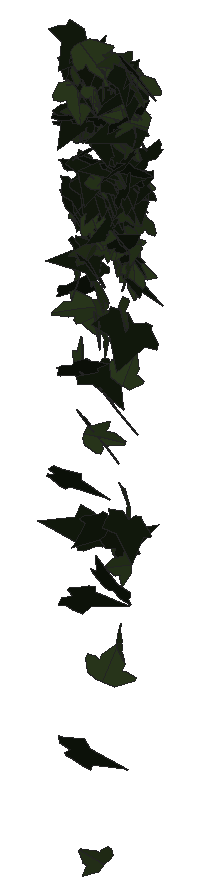
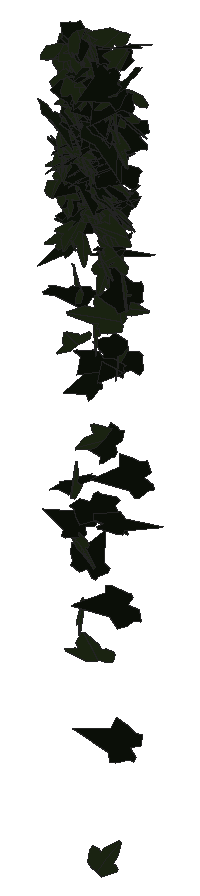
# SketchUp Ruby script. Lengths in inches.
U = 1.inch
M = Sketchup.active_model
def pt(a) = Geom::Point3d.new(a.map { |v| v * U })
def face(e, loops, mat)
  f = e.add_face(loops[0].map { |a| pt(a) })
  loops[1..].each { |l| e.add_face(l.map { |a| pt(a) }).erase! }
  f.material = f.back_material = mat if mat
  f
end
# faces: each face lists its corners as indices into pts; further lists are holes
def faces(e, pts, list, mat = nil) = list.each { |f| face(e, (f[0].is_a?(Array) ? f : [f]).map { |l| l.map { |i| pts[i] } }, mat) }
# xy, xz, yz: faces in a plane at the given z, y or x. An outline is a flat list of corners, or four numbers for a rectangle; further outlines are holes
def ring(l) = l.size == 4 ? [[l[0], l[1]], [l[2], l[1]], [l[2], l[3]], [l[0], l[3]]] : l.each_slice(2).to_a
def flat(e, list, mat, &to3) = list.each { |f| face(e, (f[0].is_a?(Array) ? f : [f]).map { |l| ring(l).map { |u, v| to3.(u, v) } }, mat) }
def xy(e, z, list, mat = nil) = flat(e, list, mat) { |x, y| [x, y, z] }
def xz(e, y, list, mat = nil) = flat(e, list, mat) { |x, z| [x, y, z] }
def yz(e, x, list, mat = nil) = flat(e, list, mat) { |y, z| [x, y, z] }
def lines(e, pts, list) = list.each { |a, b| e.add_line(pt(pts[a]), pt(pts[b])) }
# prism: a flat outline (further loops are holes) pulled along v
def prism(e, loops, v, mat = nil)
  f = face(e, loops, mat); d = Geom::Vector3d.new(v.map { |x| x * U })
  f.pushpull(f.normal.samedirection?(d) ? d.length : -d.length)
end
def box(e, o, s, mat = nil) = prism(e, [[o, [o[0] + s[0], o[1], o[2]], [o[0] + s[0], o[1] + s[1], o[2]], [o[0], o[1] + s[1], o[2]]]], [0, 0, s[2]], mat)
def at(x, y, z, deg = 0) = Geom::Transformation.translation(pt([x, y, z])) * Geom::Transformation.rotation(ORIGIN, Z_AXIS, deg.degrees)
def axes(o, x, y, z) = Geom::Transformation.new([*x, 0, *y, 0, *z, 0, *pt(o).to_a, 1])
def part(name) = M.definitions.add(name)
# library, detail: a bought-in or finely detailed component or shape, given as its bounding box
def library(name, o, s) = part(name).tap { |d| box(d.entities, o, s) }
def detail(e, o, s) = box(e.add_group.entities, o, s)
def put(e, d, t, mat = nil) = e.add_instance(d, t).tap { |i| i.material = mat if mat }
def group(e, t, mat = nil) = e.add_group.tap { |g| g.transformation = t; g.material = mat if mat }.entities
root = M.entities
M.materials.add("1026 AP 7946 SUNNY SIDE UP").color = [254, 231, 186]
M.materials.add("efeu1").color = [18, 25, 13]
M.materials.add("efeu2").color = [43, 57, 29]
c1 = part("ivyleaf_10")
p = [[0,0.5,-0.03],[-0.0625,2.02,-0.43],[-0.19,2.01,-0.46],[-0.54,1.05,-0.29],[-0.52,0.625,-0.18],[-0.83,0.76,-0.28],
  [-1.16,0.64,-0.33],[-1.15,0.33,-0.24],[-0.77,-0.39,0.02],[-0.3,-0.51,0.16],[0.04,-0.48,0.23],[-0.02,2.01,-0.4375],
  [-0.06,2.01,-0.43],[0.04,-0.49,0.23],[0.67,-0.49,0.14],[1.38,0.36,-0.2],[1.375,0.51,-0.24],[0.81,0.65,-0.19],
  [0.62,0.59,-0.15],[0.6,1.09,-0.28],[0.5,1.23,-0.31]]
faces(c1.entities,p,[[0,1,2,3,4,5,6,7,8,9,10],[11,12,0,13,14,15,16,17,18,19,20]],"efeu2")
c2 = part("ivyleaf_9")
p = [[1.54,2.16,1.25],[1.36,2.04,1.19],[-0.21,0.99,0.68],[-0.71,1.11,0.82],[-0.85,0.86,0.67],[-0.8,0.17,0.21],
  [-0.9,-0.01,0.1],[-0.67,-0.16,-0.02],[-0.08,-0.08,-0.05],[-0.03,-0.6,-0.4],[0.65,-0.88,-0.66],[0.83,-0.6,-0.49],
  [1.29,-0.42,-0.43],[1.8125,-0.07,-0.26],[1.21,0.44,0.15]]
faces(c2.entities,p,[[0,1,2,3,4,5,6,7,8,9,10,11,12,13,14]],"efeu1")
put(root,c1,axes([113.11,212.68,263.1],[0.14339,-0.21854,-0.11555],[-0.02528,0.11276,-0.24183],[0.38453,0.08891,0.02719]),"1026 AP 7946 SUNNY SIDE UP")
put(root,c1,axes([113.16,212.9,266.08],[0.28745,-0.13177,-0.11438],[-0.11976,0.0822,-0.23077],[0.24219,0.19704,0.02164]),"1026 AP 7946 SUNNY SIDE UP")
put(root,c1,axes([113.23,212.76,262.51],[-0.08031,-0.00401,0.24324],[-0.13938,-0.2236,-0.02498],[0.3442,-0.09148,0.04664]),"1026 AP 7946 SUNNY SIDE UP")
put(root,c2,axes([112.91,212.79,267.24],[0.15405,-0.23556,0.00086],[-0.00345,-0.00327,-0.26283],[0.3704,0.09794,-0.00281]),"1026 AP 7946 SUNNY SIDE UP")
put(root,c2,axes([112.79,212.7,266.14],[0.27707,-0.02474,0.18756],[0.28605,0.06019,-0.17247],[-0.04208,0.24622,0.06254]),"1026 AP 7946 SUNNY SIDE UP")
put(root,c2,axes([113.15,212.73,266.41],[-0.35367,-0.0146,-0.10812],[0.16648,-0.03342,-0.22934],[-0.00163,-0.24591,0.03612]),"1026 AP 7946 SUNNY SIDE UP")
put(root,c2,axes([112.97,212.71,262.75],[0.24374,0.17951,0.06208],[-0.08387,-0.03196,0.24337],[0.28515,-0.16284,0.01852]),"1026 AP 7946 SUNNY SIDE UP")
put(root,c2,axes([112.83,212.51,259.08],[0.31998,-0.00455,0.13415],[0.204,-0.01583,-0.20949],[0.01944,0.24109,-0.00981]),"1026 AP 7946 SUNNY SIDE UP")
put(root,c1,axes([113.1875,212.68,261.35],[-0.03383,0.16262,-0.1746],[-0.02819,0.16949,0.16995],[0.36931,0.02784,-0.00302]),"1026 AP 7946 SUNNY SIDE UP")
put(root,c2,axes([113.16,212.82,267.87],[-0.27569,-0.18209,0.07565],[0.01248,-0.10621,-0.24894],[0.30908,-0.15813,0.07752]),"1026 AP 7946 SUNNY SIDE UP")
put(root,c2,axes([112.98,212.79,264.84],[0.09227,-0.24022,0.02704],[0.00198,-0.02811,-0.25485],[0.3802,0.05844,-0.00524]),"1026 AP 7946 SUNNY SIDE UP")
put(root,c1,axes([113.11,212.9,266.38],[0.14453,-0.21357,0.09729],[0.10596,-0.07425,-0.23795],[0.35238,0.10992,0.03165]),"1026 AP 7946 SUNNY SIDE UP")
put(root,c2,axes([113.46,212.74,258.04],[-0.20765,0.00261,0.22035],[-0.33108,-0.04579,-0.13363],[0.05915,-0.24716,0.02559]),"1026 AP 7946 SUNNY SIDE UP")
put(root,c1,axes([112.89,213.01,264.22],[0.07986,0.02033,0.23675],[0.36249,-0.01001,-0.05166],[0.00854,0.23503,-0.02129]),"1026 AP 7946 SUNNY SIDE UP")
put(root,c2,axes([112.98,212.7,264.55],[0.15702,-0.21785,0.07841],[0.03027,-0.07613,-0.24693],[0.36223,0.10079,-0.01335]),"1026 AP 7946 SUNNY SIDE UP")
put(root,c2,axes([113.44,212.88,264.79],[-0.16271,0.20616,0.07975],[-0.13387,0.0401,-0.2305],[-0.31864,-0.12212,0.05612]),"1026 AP 7946 SUNNY SIDE UP")
put(root,c2,axes([112.97,212.79,256.57],[0.08033,0.09459,-0.23035],[0.13195,0.20812,0.11141],[0.35906,-0.09764,0.01059]),"1026 AP 7946 SUNNY SIDE UP")
put(root,c1,axes([112.95,212.97,264.47],[0.23372,-0.06389,-0.18259],[0.28207,-0.01951,0.16245],[-0.08877,-0.23021,0.03545]),"1026 AP 7946 SUNNY SIDE UP")
put(root,c1,axes([113.15,212.92,266.87],[0.02845,0.25366,0.00702],[-0.0002,0.00539,-0.26195],[-0.39894,0.01809,0.00063]),"1026 AP 7946 SUNNY SIDE UP")
put(root,c2,axes([113.38,212.6875,264.37],[0.02959,0.08398,0.26584],[-0.10849,0.25116,-0.0777],[-0.41194,-0.06012,0.03956]),"1026 AP 7946 SUNNY SIDE UP")
put(root,c2,axes([113.19,212.9375,264.66],[-0.15171,-0.21094,0.06917],[-0.00318,-0.07369,-0.23769],[0.34865,-0.09246,0.02793]),"1026 AP 7946 SUNNY SIDE UP")
put(root,c2,axes([113.17,212.8125,266.98],[0.25403,0.19503,0.04641],[0.05454,0.0283,-0.26059],[-0.30959,0.16502,-0.00783]),"1026 AP 7946 SUNNY SIDE UP")
put(root,c1,axes([113.1,212.65,266.89],[0.39992,0.05938,0.06721],[0.10794,-0.0098,-0.26794],[-0.0865,0.2623,-0.02361]),"1026 AP 7946 SUNNY SIDE UP")
put(root,c2,axes([112.99,213.12,259.95],[0.24103,-0.18315,0.08435],[0.07013,-0.0707,-0.24622],[0.30826,0.1593,-0.00994]),"1026 AP 7946 SUNNY SIDE UP")
put(root,c1,axes([113.3,212.78,266.48],[-0.32134,-0.14247,0.01436],[-0.0011,-0.0247,-0.25598],[0.22522,-0.2034,0.01923]),"1026 AP 7946 SUNNY SIDE UP")
put(root,c2,axes([113.08,212.6875,265.43],[0.34831,0.10374,0.05498],[0.08308,0.01148,-0.25163],[-0.16307,0.22743,-0.01077]),"1026 AP 7946 SUNNY SIDE UP")
put(root,c2,axes([113.16,212.86,267.14],[0.16056,0.15054,0.22448],[0.19108,0.17984,-0.18634],[-0.36878,0.15872,0.00118]),"1026 AP 7946 SUNNY SIDE UP")
put(root,c1,axes([113.37,213.02,251.24],[-0.11316,-0.14568,-0.20001],[-0.16278,-0.16379,0.1659],[-0.34406,0.12541,-0.0127]),"1026 AP 7946 SUNNY SIDE UP")
put(root,c2,axes([113.51,212.76,263.55],[-0.2734,-0.02419,0.17293],[-0.2298,-0.10097,-0.17139],[0.13573,-0.21969,0.05816]),"1026 AP 7946 SUNNY SIDE UP")
put(root,c1,axes([113.27,212.54,267.52],[0.03286,0.20384,0.17846],[-0.05247,0.17324,-0.20623],[-0.41615,-0.00575,0.04009]),"1026 AP 7946 SUNNY SIDE UP")
put(root,c2,axes([113.47,212.88,266.04],[-0.00762,0.24899,0.03723],[-0.09424,0.03258,-0.24913],[-0.3839,-0.01294,0.06042]),"1026 AP 7946 SUNNY SIDE UP")
put(root,c2,axes([113.125,212.71,263.75],[0.22541,-0.19566,-0.01982],[-0.02659,0.01007,-0.24969],[0.30782,0.14415,-0.00705]),"1026 AP 7946 SUNNY SIDE UP")
put(root,c1,axes([113.08,212.95,263.67],[0.2639,-0.02544,0.16899],[0.25765,-0.01316,-0.17474],[0.04311,0.23441,0.00992]),"1026 AP 7946 SUNNY SIDE UP")
put(root,c2,axes([113.46,212.7,265.86],[-0.03787,0.2489,-0.01265],[-0.00255,-0.01391,-0.25768],[-0.39196,-0.02396,0.0029]),"1026 AP 7946 SUNNY SIDE UP")
put(root,c2,axes([113.25,212.42,261.47],[0.25901,0.181,0.05835],[0.07257,0.03311,-0.25164],[-0.28875,0.17067,-0.01091]),"1026 AP 7946 SUNNY SIDE UP")
put(root,c1,axes([113.41,212.65,263.8],[-0.07233,-0.22693,0.05058],[-0.00303,-0.05099,-0.23869],[0.3655,-0.04533,0.00803]),"1026 AP 7946 SUNNY SIDE UP")
put(root,c1,axes([113.31,212.85,264.42],[-0.36001,-0.06725,-0.05867],[0.12713,-0.09934,-0.21603],[0.05415,-0.2139,0.11713]),"1026 AP 7946 SUNNY SIDE UP")
put(root,c1,axes([113.32,212.8125,266.36],[-0.02745,0.07669,-0.25279],[0.01927,-0.24585,-0.08135],[-0.40443,-0.01692,0.01328]),"1026 AP 7946 SUNNY SIDE UP")
put(root,c1,axes([113.42,212.85,265],[-0.36384,-0.07137,0.01785],[0.01596,-0.08896,-0.23302],[0.11453,-0.21434,0.08916]),"1026 AP 7946 SUNNY SIDE UP")
put(root,c2,axes([113.33,212.6,267.28],[-0.09798,-0.08593,0.25551],[0.2938,0.16522,0.10809],[-0.2909,0.19581,0.02311]),"1026 AP 7946 SUNNY SIDE UP")
put(root,c2,axes([113.35,212.9,265.01],[-0.28616,-0.08708,-0.14489],[0.2253,0.02007,-0.2044],[0.12866,-0.22882,0.03566]),"1026 AP 7946 SUNNY SIDE UP")
put(root,c2,axes([113.07,212.61,253.5625],[0.2214,-0.03551,0.22121],[0.31491,-0.07961,-0.14918],[0.13479,0.24431,-0.01485]),"1026 AP 7946 SUNNY SIDE UP")
put(root,c1,axes([113.48,212.94,265.11],[-0.03085,-0.24314,0.00966],[-0.00318,-0.01063,-0.25135],[0.38267,-0.01969,-0.00131]),"1026 AP 7946 SUNNY SIDE UP")
put(root,c1,axes([113.39,212.91,263.47],[0.23129,-0.17155,0.07394],[0.07233,-0.05639,-0.23312],[0.28393,0.15411,-0.00085]),"1026 AP 7946 SUNNY SIDE UP")
put(root,c1,axes([113.3125,212.89,259.88],[0.05431,0.06055,0.23759],[0.12432,0.21657,-0.06961],[-0.35316,0.08555,0.01203]),"1026 AP 7946 SUNNY SIDE UP")
put(root,c2,axes([113.55,212.78,266.6],[0.22399,0.15272,-0.1568],[-0.17696,-0.10415,-0.21556],[-0.29031,0.18132,0.01042]),"1026 AP 7946 SUNNY SIDE UP")
put(root,c2,axes([113.53,212.86,265.09],[-0.19793,0.10736,-0.18339],[0.15727,-0.15195,-0.16759],[-0.28748,-0.15704,0.03458]),"1026 AP 7946 SUNNY SIDE UP")
put(root,c2,axes([113.42,212.78,265.4],[-0.12178,-0.23438,0.06477],[-0.01196,-0.06502,-0.25433],[0.38192,-0.07677,0.01269]),"1026 AP 7946 SUNNY SIDE UP")
put(root,c2,axes([113.37,212.68,266.31],[0.34939,0.12801,0.00971],[0.02646,-0.01183,-0.26355],[-0.20001,0.22206,-0.0179]),"1026 AP 7946 SUNNY SIDE UP")
put(root,c1,axes([113.38,212.95,264.79],[0.31388,-0.09748,0.09918],[0.15047,-0.02389,-0.22817],[0.15502,0.22057,0.02067]),"1026 AP 7946 SUNNY SIDE UP")
put(root,c2,axes([113.54,212.79,265.05],[-0.31747,-0.10704,-0.08393],[0.14402,-0.00323,-0.23121],[0.15412,-0.21747,0.04316]),"1026 AP 7946 SUNNY SIDE UP")
put(root,c1,axes([113.5625,212.68,263.1],[-0.26868,0.17235,0.00308],[-0.02039,-0.01003,-0.24952],[-0.27025,-0.17059,0.01577]),"1026 AP 7946 SUNNY SIDE UP")
put(root,c1,axes([113.24,212.89,262.34],[0.06545,0.02044,0.28839],[0.39055,0.12888,-0.04701],[-0.20518,0.25184,0.00251]),"1026 AP 7946 SUNNY SIDE UP")
put(root,c1,axes([113.56,212.8,267.05],[-0.15315,0.19436,-0.13373],[-0.00695,-0.14327,-0.21657],[-0.36841,-0.07809,0.05968]),"1026 AP 7946 SUNNY SIDE UP")
put(root,c1,axes([113.52,212.81,267.05],[0.24578,0.19921,-0.01645],[0.00052,-0.02196,-0.2606],[-0.31439,0.1557,-0.01329]),"1026 AP 7946 SUNNY SIDE UP")
put(root,c1,axes([113.44,212.52,267.87],[0.17244,0.21559,0.12765],[0.11529,0.09997,-0.24792],[-0.37261,0.1307,-0.01763]),"1026 AP 7946 SUNNY SIDE UP")
put(root,c2,axes([113.54,212.8125,266.21],[0.35864,-0.0202,-0.10636],[-0.16272,-0.00034,-0.23572],[0.02872,0.25031,-0.00743]),"1026 AP 7946 SUNNY SIDE UP")
put(root,c2,axes([113.75,212.76,258.36],[0.02569,0.09211,-0.24125],[-0.04923,-0.23264,-0.09766],[-0.39339,0.03513,-0.00353]),"1026 AP 7946 SUNNY SIDE UP")
put(root,c2,axes([113.55,212.9375,265.17],[-0.09619,-0.23516,0.02652],[-0.00148,-0.02773,-0.2504],[0.3722,-0.06089,0.00586]),"1026 AP 7946 SUNNY SIDE UP")
put(root,c1,axes([113.75,212.73,264.03],[0.22627,-0.14545,-0.12574],[-0.15163,0.07474,-0.20987],[0.25622,0.17267,-0.01316]),"1026 AP 7946 SUNNY SIDE UP")
put(root,c1,axes([113.56,212.67,262.4],[-0.09415,0.15877,-0.17054],[0.07736,-0.15917,-0.17558],[-0.35331,-0.07716,0.007]),"1026 AP 7946 SUNNY SIDE UP")
put(root,c2,axes([113.75,212.84,265.09],[0.07144,0.23633,-0.03288],[-0.00345,-0.03345,-0.24808],[-0.37525,0.0453,-0.00398]),"1026 AP 7946 SUNNY SIDE UP")
put(root,c2,axes([113.51,212.78,261.39],[-0.12223,-0.12418,-0.20028],[0.22183,0.1358,-0.14721],[0.28581,-0.1585,0.02861]),"1026 AP 7946 SUNNY SIDE UP")
put(root,c1,axes([113.72,212.73,261.98],[0.16248,-0.18346,-0.14607],[-0.02925,0.14707,-0.21069],[0.36241,0.09412,0.04848]),"1026 AP 7946 SUNNY SIDE UP")
put(root,c1,axes([113.6,212.53,264.5],[0.13535,0.2368,0.0401],[0.03486,0.0319,-0.25918],[-0.37539,0.08834,-0.00961]),"1026 AP 7946 SUNNY SIDE UP")
put(root,c1,axes([113.71,212.91,264.65],[0.18507,-0.20631,0.01557],[-0.00186,-0.0194,-0.24456],[0.3254,0.11722,-0.01025]),"1026 AP 7946 SUNNY SIDE UP")
put(root,c1,axes([113.72,212.83,267.65],[0.19672,-0.23128,-0.00934],[0.00799,0.01156,-0.27063],[0.36379,0.12482,0.011]),"1026 AP 7946 SUNNY SIDE UP")
put(root,c2,axes([113.65,212.62,266.14],[0.23679,-0.08856,-0.18939],[-0.14171,0.17548,-0.16256],[0.28707,0.15967,0.07597]),"1026 AP 7946 SUNNY SIDE UP")
put(root,c1,axes([113.72,212.61,264.22],[0.29826,-0.16998,0.04957],[-0.02971,0.05208,0.26136],[-0.27661,-0.18888,0.02537]),"1026 AP 7946 SUNNY SIDE UP")
put(root,c1,axes([113.75,212.95,265.3125],[0.21138,-0.20333,0.02658],[0.03209,-0.0188,-0.25113],[0.32091,0.13581,0.00761]),"1026 AP 7946 SUNNY SIDE UP")
put(root,c1,axes([113.57,212.89,265.08],[0.30301,0.02641,0.15759],[0.24281,-0.01007,-0.19886],[-0.02261,0.24574,-0.02362]),"1026 AP 7946 SUNNY SIDE UP")
put(root,c1,axes([113.69,212.76,255.27],[0.38128,0.07194,-0.07632],[0.10061,0.04506,0.25966],[0.12803,-0.24964,0.02324]),"1026 AP 7946 SUNNY SIDE UP")
put(root,c2,axes([113.65,212.87,267],[-0.16687,-0.17968,-0.14989],[0.19049,0.09187,-0.20884],[0.30846,-0.15393,0.04788]),"1026 AP 7946 SUNNY SIDE UP")
put(root,c1,axes([113.88,212.93,263.75],[-0.29479,0.14058,0.04458],[-0.10442,-0.01972,-0.23485],[-0.20597,-0.19122,0.05525]),"1026 AP 7946 SUNNY SIDE UP")
put(root,c2,axes([113.83,212.78,257.03],[0.26502,-0.1448,0.12277],[-0.11692,0.09669,0.22836],[-0.2716,-0.18291,0.02149]),"1026 AP 7946 SUNNY SIDE UP")
put(root,c1,axes([113.86,212.86,267.36],[0.23774,-0.18729,-0.08885],[-0.07111,0.07287,-0.24733],[0.31561,0.1575,0.0112]),"1026 AP 7946 SUNNY SIDE UP")
put(root,c2,axes([113.67,212.94,265.03],[0.05691,-0.2404,0.01658],[0.00133,-0.01753,-0.25054],[0.379,0.03616,-0.00161]),"1026 AP 7946 SUNNY SIDE UP")
put(root,c2,axes([113.77,212.79,267.38],[-0.3007,-0.06196,-0.17097],[0.26485,0.0104,-0.20432],[0.0846,-0.25277,0.03193]),"1026 AP 7946 SUNNY SIDE UP")
put(root,c1,axes([113.81,212.81,266.78],[0.37204,-0.09439,-0.03052],[0.00008,0.07563,-0.25194],[0.15531,0.22607,0.07324]),"1026 AP 7946 SUNNY SIDE UP")
put(root,c2,axes([113.75,212.92,265.07],[-0.0422,-0.23813,0.05112],[0.0041,-0.05156,-0.24703],[0.38289,-0.02569,0.00828]),"1026 AP 7946 SUNNY SIDE UP")
put(root,c1,axes([113.85,212.9,265.14],[0.3407,-0.10555,-0.0133],[-0.03177,-0.01346,-0.24744],[0.16405,0.21661,-0.02029]),"1026 AP 7946 SUNNY SIDE UP")
put(root,c2,axes([113.74,212.9,265.3],[-0.02911,-0.24211,0.04988],[0.00429,-0.05013,-0.25036],[0.38864,-0.01758,0.0065]),"1026 AP 7946 SUNNY SIDE UP")
put(root,c1,axes([113.87,212.75,266.68],[-0.12507,0.23994,-0.03717],[-0.05429,-0.05017,-0.25597],[-0.37798,-0.07219,0.04906]),"1026 AP 7946 SUNNY SIDE UP")
put(root,c1,axes([113.79,212.83,267.38],[0.16912,-0.22218,0.0669],[0.12241,-0.03413,-0.24849],[0.34337,0.1216,0.05564]),"1026 AP 7946 SUNNY SIDE UP")
put(root,c2,axes([113.66,212.78,260.89],[0.30423,-0.14553,0.01707],[0.00407,-0.02541,-0.24882],[0.23043,0.19259,-0.01814]),"1026 AP 7946 SUNNY SIDE UP")
put(root,c1,axes([114.05,212.84,257.56],[0.1687,-0.13157,-0.18188],[-0.20295,0.12051,-0.17335],[0.27933,0.16702,-0.0161]),"1026 AP 7946 SUNNY SIDE UP")
put(root,c1,axes([113.83,212.61,265.375],[-0.27913,-0.15522,-0.06399],[0.15523,-0.02561,-0.22809],[0.21154,-0.18603,0.08293]),"1026 AP 7946 SUNNY SIDE UP")
put(root,c2,axes([113.74,212.88,265.13],[0.38046,0.02026,0.00087],[0.0015,-0.00267,-0.25014],[-0.03183,0.24195,-0.00141]),"1026 AP 7946 SUNNY SIDE UP")
put(root,c1,axes([113.97,212.89,266.89],[-0.22344,-0.20784,0.02095],[-0.00511,-0.02382,-0.25928],[0.32852,-0.14174,0.01022]),"1026 AP 7946 SUNNY SIDE UP")
put(root,c1,axes([113.97,212.87,267.54],[-0.29708,-0.17229,0.0156],[-0.00022,-0.02372,-0.26294],[0.2721,-0.18813,0.01682]),"1026 AP 7946 SUNNY SIDE UP")
put(root,c1,axes([113.96,212.84,267.76],[-0.10829,-0.25077,0.0349],[0.00499,-0.03743,-0.2678],[0.39817,-0.06773,0.01285]),"1026 AP 7946 SUNNY SIDE UP")
put(root,c1,axes([113.97,212.85,265],[0.04997,-0.24704,-0.01032],[0.02171,0.01045,-0.25607],[0.38808,0.03123,0.01566]),"1026 AP 7946 SUNNY SIDE UP")
put(root,c1,axes([114.08,212.66,256.05],[-0.09158,0.09617,0.22311],[-0.20622,0.17198,-0.1143],[-0.30938,-0.14311,0.01014]),"1026 AP 7946 SUNNY SIDE UP")
put(root,c2,axes([113.75,212.88,267.35],[0.21903,-0.21769,-0.00033],[0.00789,0.00212,-0.26618],[0.34221,0.13928,0.00635]),"1026 AP 7946 SUNNY SIDE UP")
put(root,c1,axes([114.08,212.98,265.48],[0.32508,-0.0152,-0.13334],[-0.20478,-0.02224,-0.21188],[0.0016,0.24286,-0.02631]),"1026 AP 7946 SUNNY SIDE UP")
put(root,c2,axes([114.05,212.81,264.5],[-0.006,-0.03065,-0.25099],[0.06289,-0.24031,0.02911],[-0.38067,-0.03922,0.00877]),"1026 AP 7946 SUNNY SIDE UP")
put(root,c1,axes([113.96,212.93,265.38],[0.36328,-0.08052,0.00464],[-0.00362,-0.02163,-0.25123],[0.12679,0.23007,-0.02047]),"1026 AP 7946 SUNNY SIDE UP")
put(root,c1,axes([113.96,213.04,258.66],[-0.21844,0.16878,0.10891],[0.11663,-0.07452,0.22457],[0.28976,0.15723,-0.00828]),"1026 AP 7946 SUNNY SIDE UP")
put(root,c2,axes([113.93,212.77,265.29],[0.36216,0.03088,-0.08054],[-0.12201,-0.0109,-0.23946],[-0.05149,0.24304,0.00095]),"1026 AP 7946 SUNNY SIDE UP")
put(root,c2,axes([114.22,212.75,267.54],[-0.27463,0.1899,-0.02259],[0.00532,-0.02807,-0.26542],[-0.30074,-0.17392,0.01593]),"1026 AP 7946 SUNNY SIDE UP")
put(root,c1,axes([114.03,212.62,265.53],[-0.2787,0.17129,-0.01264],[-0.00436,-0.02187,-0.25341],[-0.27011,-0.17639,0.01713]),"1026 AP 7946 SUNNY SIDE UP")
put(root,c2,axes([113.83,212.82,266.74],[0.25753,-0.19658,-0.01146],[0.00358,0.01491,-0.26325],[0.30948,0.16341,0.01258]),"1026 AP 7946 SUNNY SIDE UP")
put(root,c1,axes([113.98,212.81,267.48],[0.19384,0.22404,-0.01064],[0.00952,-0.01655,-0.26318],[-0.35263,0.12271,-0.01295]),"1026 AP 7946 SUNNY SIDE UP")
put(root,c2,axes([114.34,212.71,265.73],[-0.32693,0.01245,0.134],[-0.20523,-0.02846,-0.2124],[0.00727,-0.24356,0.03022]),"1026 AP 7946 SUNNY SIDE UP")
put(root,c2,axes([113.89,212.84,257.875],[-0.02377,0.00946,0.25068],[0.34875,0.10105,0.01074],[-0.15786,0.22181,-0.01402]),"1026 AP 7946 SUNNY SIDE UP")
put(root,c1,axes([114.02,212.91,263.95],[0.08009,0.21655,0.09432],[-0.00634,0.09323,-0.22736],[-0.36888,0.04542,0.02439]),"1026 AP 7946 SUNNY SIDE UP")
put(root,c2,axes([114.05,212.9,265.3],[-0.23745,-0.19248,-0.01407],[0.06032,-0.01433,-0.2489],[0.29724,-0.15085,0.03927]),"1026 AP 7946 SUNNY SIDE UP")
put(root,c1,axes([114.02,212.75,264.28],[0.37471,0.01882,0.00065],[0.00336,-0.02044,-0.24547],[-0.02941,0.23742,-0.01977]),"1026 AP 7946 SUNNY SIDE UP")
put(root,c1,axes([113.81,212.66,267.02],[-0.14065,-0.03115,-0.24672],[0.35183,-0.10634,-0.07252],[-0.14219,-0.2323,0.06461]),"1026 AP 7946 SUNNY SIDE UP")
put(root,c1,axes([113.97,212.71,266.33],[-0.34468,-0.06464,-0.1299],[0.20791,-0.01164,-0.23139],[0.07868,-0.25243,0.04236]),"1026 AP 7946 SUNNY SIDE UP")
put(root,c2,axes([113.96,212.82,265.35],[0.02268,-0.24343,-0.06645],[-0.00809,0.06293,-0.25085],[0.39535,0.01525,-0.00132]),"1026 AP 7946 SUNNY SIDE UP")
put(root,c2,axes([113.87,212.63,264],[0.41306,0.02182,-0.03605],[0.04391,0.07292,0.26231],[0.04794,-0.2548,0.07036]),"1026 AP 7946 SUNNY SIDE UP")
put(root,c2,axes([114.08,212.93,265.43],[-0.11071,-0.2358,0.00527],[0.0103,-0.00869,-0.2534],[0.37076,-0.07017,0.00861]),"1026 AP 7946 SUNNY SIDE UP")
put(root,c1,axes([114.18,212.98,265.36],[-0.1419,-0.2255,-0.01609],[0.03497,0.0065,-0.24948],[0.35356,-0.09114,0.01822]),"1026 AP 7946 SUNNY SIDE UP")
put(root,c2,axes([114.37,212.6875,266.59],[-0.3825,-0.0193,0.06172],[-0.08814,-0.04326,-0.24865],[0.04536,-0.24679,0.03727]),"1026 AP 7946 SUNNY SIDE UP")
put(root,c2,axes([114.31,212.44,265.29],[-0.02327,0.09052,0.25441],[-0.03246,0.24566,-0.0928],[-0.41153,-0.02449,-0.00707]),"1026 AP 7946 SUNNY SIDE UP")
put(root,c2,axes([114.29,212.66,267.37],[-0.3398,0.09548,-0.10602],[0.11998,-0.07985,-0.24058],[-0.18604,-0.22589,0.03851]),"1026 AP 7946 SUNNY SIDE UP")
put(root,c2,axes([113.98,212.82,267.74],[0.37481,-0.10139,-0.01121],[-0.03062,-0.01956,-0.26566],[0.1573,0.23778,-0.02499]),"1026 AP 7946 SUNNY SIDE UP")
put(root,c2,axes([113.99,212.84,264.21],[0.20036,-0.20579,0.0418],[0.01503,-0.04309,-0.24917],[0.32984,0.12697,-0.01404]),"1026 AP 7946 SUNNY SIDE UP")
put(root,c1,axes([114.02,212.82,262.67],[-0.0065,-0.00907,-0.29551],[0.15761,-0.2688,0.00569],[-0.42276,-0.10007,0.00666]),"1026 AP 7946 SUNNY SIDE UP")
put(root,c1,axes([114.34,212.93,264.64],[-0.34113,0.05524,0.08937],[-0.14688,-0.02284,-0.22664],[-0.06665,-0.23241,0.04207]),"1026 AP 7946 SUNNY SIDE UP")
put(root,c1,axes([114.22,212.98,265.48],[0.08652,-0.21416,-0.10811],[0.02023,0.10899,-0.22414],[0.37361,0.04369,0.03717]),"1026 AP 7946 SUNNY SIDE UP")
put(root,c1,axes([114.17,212.69,261.44],[0.16738,0.15102,-0.16052],[0.07191,0.15499,0.18683],[0.33453,-0.10888,0.04015]),"1026 AP 7946 SUNNY SIDE UP")
put(root,c1,axes([114.15,212.92,265.29],[0.18035,0.21119,-0.0123],[0.00631,-0.01712,-0.24739],[-0.33266,0.11417,-0.01136]),"1026 AP 7946 SUNNY SIDE UP")
put(root,c1,axes([114.35,212.65,266.41],[0.12934,-0.18053,-0.1993],[-0.13722,0.17161,-0.20328],[0.39153,0.11978,-0.00541]),"1026 AP 7946 SUNNY SIDE UP")
put(root,c2,axes([114.12,212.9,265.63],[-0.02667,-0.24778,0.01916],[-0.00155,-0.01998,-0.25597],[0.39087,-0.01699,0.00029]),"1026 AP 7946 SUNNY SIDE UP")
put(root,c2,axes([114.38,212.625,266.0625],[-0.27757,0.1668,-0.14048],[0.12028,-0.11757,-0.24914],[-0.31771,-0.19024,0.02841]),"1026 AP 7946 SUNNY SIDE UP")
put(root,c1,axes([114.27,212.98,265.67],[0.03132,-0.24451,-0.01868],[0.01333,0.01748,-0.25242],[0.38514,0.01928,0.01026]),"1026 AP 7946 SUNNY SIDE UP")
put(root,c2,axes([114.14,212.54,265.73],[0.3521,0.10572,-0.00379],[0.0087,-0.02169,-0.25422],[-0.16614,0.22291,-0.02134]),"1026 AP 7946 SUNNY SIDE UP")
put(root,c1,axes([114.41,212.76,266.61],[0.04095,0.12256,0.26224],[-0.12808,-0.24079,0.12696],[0.42434,-0.08451,0.01301]),"1026 AP 7946 SUNNY SIDE UP")
put(root,c1,axes([114.23,212.79,263.75],[0.1329,-0.1792,0.13802],[0.09869,-0.11961,-0.20475],[0.33869,0.10517,0.0055]),"1026 AP 7946 SUNNY SIDE UP")
put(root,c1,axes([114.44,212.6,267.48],[-0.26894,0.12564,0.1564],[-0.20551,0.07687,-0.2178],[-0.23076,-0.21489,0.01169]),"1026 AP 7946 SUNNY SIDE UP")
put(root,c2,axes([114.29,212.76,262.51],[-0.307,-0.20842,-0.0421],[0.0652,0.0154,-0.29343],[0.32717,-0.19864,0.01897]),"1026 AP 7946 SUNNY SIDE UP")
put(root,c2,axes([114.15,212.64,266.53],[0.20798,0.22429,0.09378],[-0.08547,-0.07208,0.26764],[0.37013,-0.14267,0.00911]),"1026 AP 7946 SUNNY SIDE UP")
put(root,c2,axes([114.19,212.99,265.25],[-0.01917,-0.24137,0.0164],[0.00054,-0.01732,-0.24907],[0.3805,-0.01213,0.00118]),"1026 AP 7946 SUNNY SIDE UP")
put(root,c1,axes([114.25,212.73,264.88],[-0.15176,-0.18564,-0.14919],[0.16346,0.10558,-0.21174],[0.33104,-0.13724,0.03616]),"1026 AP 7946 SUNNY SIDE UP")
put(root,c1,axes([114.34,212.87,267.4],[-0.34179,-0.14038,0.01473],[0.06358,-0.08845,-0.24803],[0.2127,-0.19913,0.09781]),"1026 AP 7946 SUNNY SIDE UP")
put(root,c2,axes([114.23,212.76,267.46],[-0.03188,-0.2501,0.06443],[-0.00463,-0.06393,-0.25886],[0.40589,-0.02037,0.00211]),"1026 AP 7946 SUNNY SIDE UP")
put(root,c1,axes([114.5,212.57,264.33],[0.14641,-0.14863,-0.19217],[-0.1872,0.14351,-0.179],[0.32377,0.15019,-0.01659]),"1026 AP 7946 SUNNY SIDE UP")
put(root,c2,axes([114.55,212.8,265.41],[-0.29094,0.15752,-0.00544],[-0.01166,-0.01822,-0.2497],[-0.24759,-0.18423,0.01816]),"1026 AP 7946 SUNNY SIDE UP")
put(root,c2,axes([114.1875,212.76,263.53],[0.30359,-0.11786,-0.10366],[-0.08182,0.10103,-0.22569],[0.22881,0.19251,0.05684]),"1026 AP 7946 SUNNY SIDE UP")
put(root,c2,axes([114.27,212.68,258.59],[-0.08067,-0.23861,-0.0284],[0.02069,0.02397,-0.25117],[0.37688,-0.05239,0.00771]),"1026 AP 7946 SUNNY SIDE UP")
put(root,c1,axes([114.3125,212.79,263.62],[0.15827,0.21556,-0.0251],[-0.01214,-0.02463,-0.24521],[-0.34112,0.10089,-0.00291]),"1026 AP 7946 SUNNY SIDE UP")
put(root,c2,axes([114.63,212.77,265.97],[-0.09173,0.2135,0.11802],[-0.09365,0.10031,-0.22565],[-0.36837,-0.07867,0.02798]),"1026 AP 7946 SUNNY SIDE UP")
